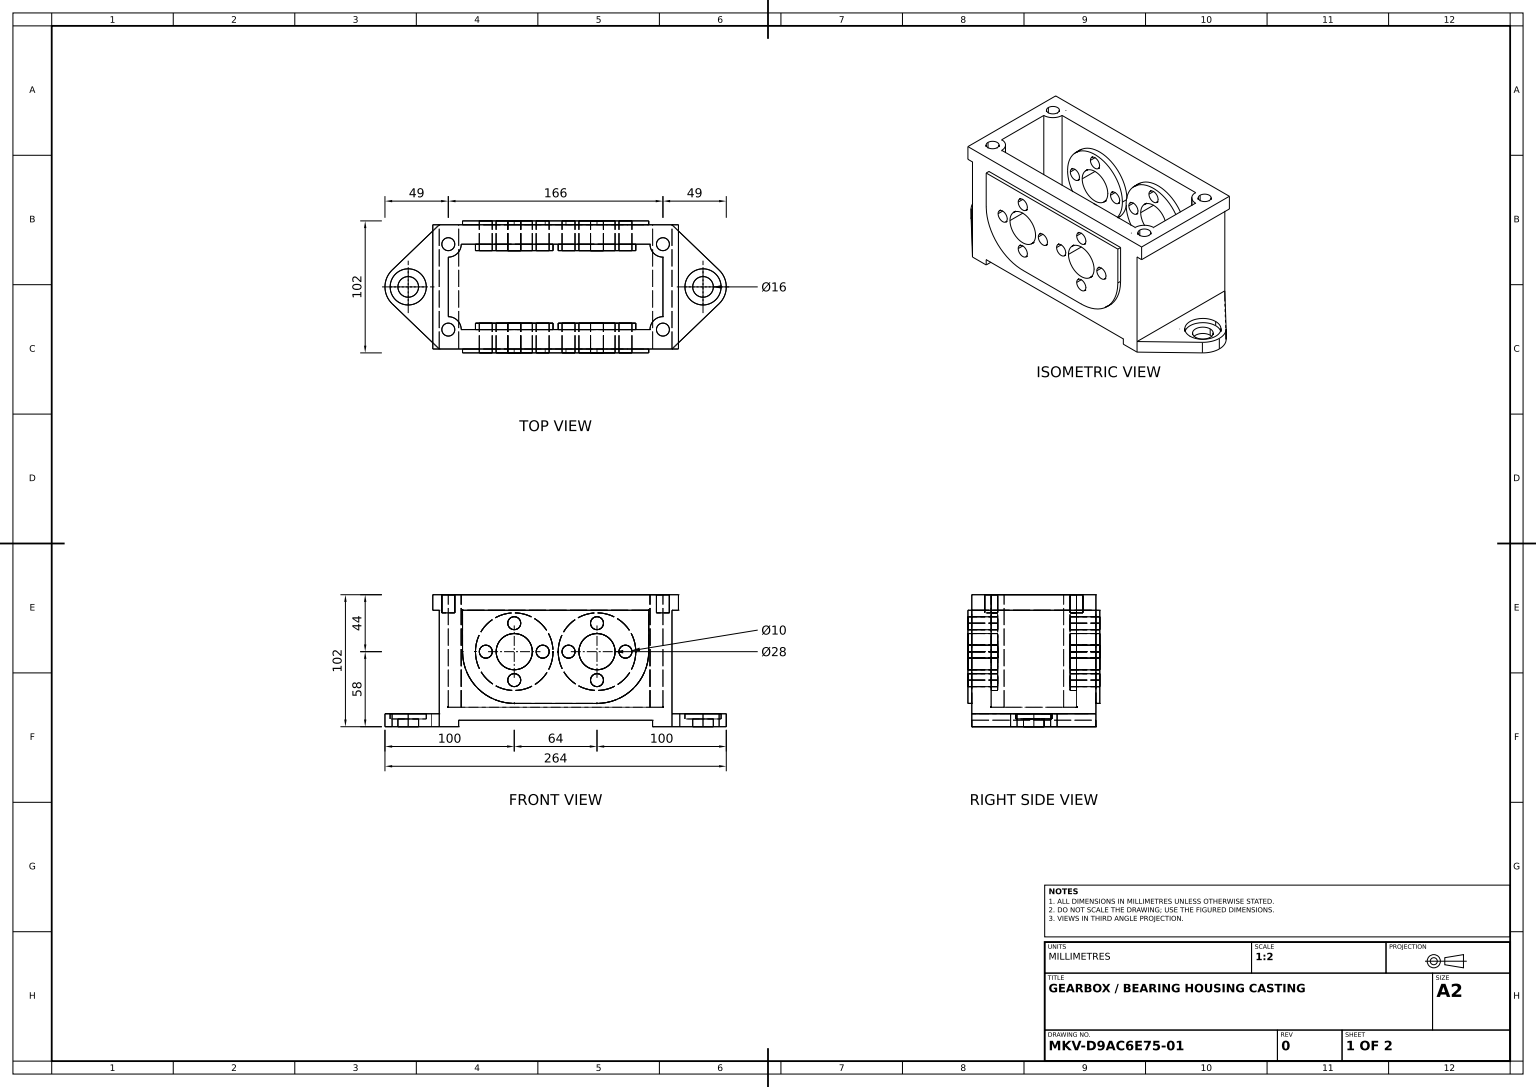
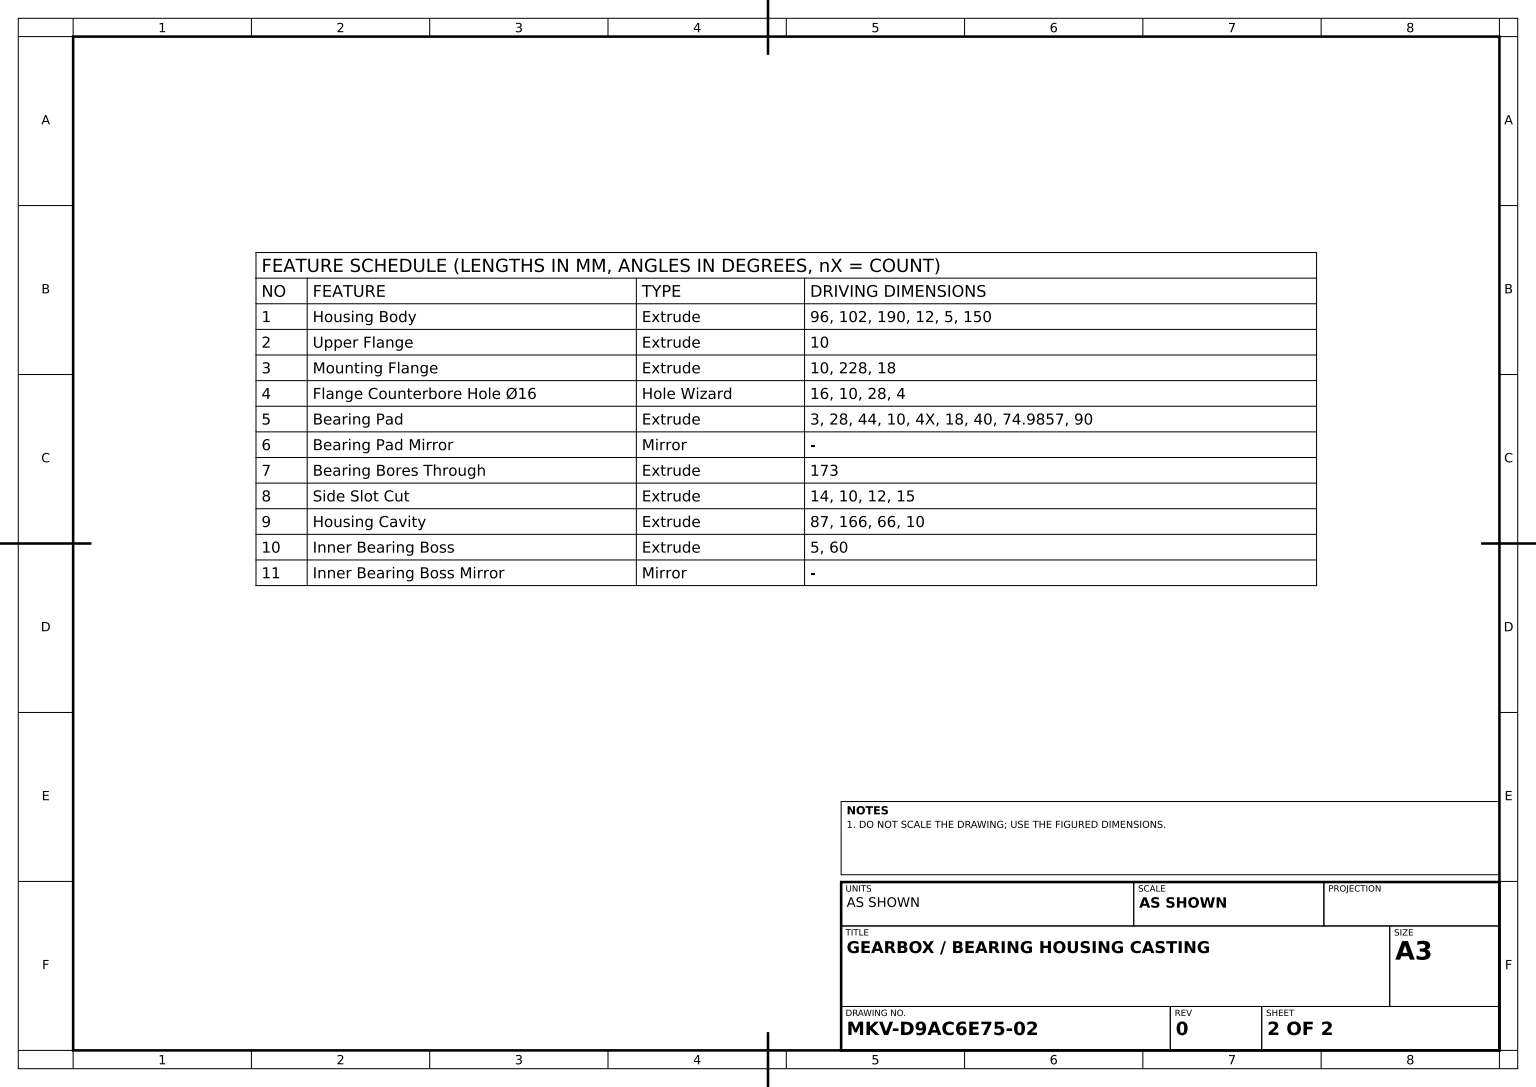
solid
v1 (75,-51,-48)
v2 (90,-51,-48)
e1 v1 v2 LINE
v3 (126.46707,-51,-12.983535)
e2 v2 v3 LINE
v4 (132,-51,0)
e3 v3 v4 CIRCLE(AX(P(114,-51,0),D(0,-1,0),D(1,0,0)),18)
v5 (126.46707,-51,12.983535)
e4 v4 v5 CIRCLE(AX(P(114,-51,0),D(0,-1,0),D(1,0,0)),18)
v6 (90,-51,48)
e5 v5 v6 LINE
v7 (75,-51,48)
e6 v7 v6 LINE
e7 v7 v1 LINE
v8 (114,-51,8)
v9 (114,-51,-8)
e8 v8 v9 CIRCLE(AX(P(114,-51,0),D(0,1,0),D(0,0,1)),8)
e9 v9 v8 CIRCLE(AX(P(114,-51,0),D(0,1,0),D(0,0,1)),8)
face PLANE(AX(P(0,-51,48),D(0,1,0),D(-1,0,0))) rev [e1 e2 e3 e4 e5 -e6 e7] [e8 e9]
v10 (78,37,33)
v11 (78,51,33)
e10 v10 v11 LINE
v12 (88,51,33)
e11 v11 v12 CIRCLE(AX(P(83,51,33),D(0,1,0),D(-1,0,0)),5)
v13 (88,37,33)
e12 v13 v12 LINE
e13 v10 v13 CIRCLE(AX(P(83,37,33),D(0,1,0),D(-1,0,0)),5)
face CYL(AX(P(83,37,33),D(0,1,0),D(-1,0,0)),5) rev [e10 e11 -e12 -e13]
v14 (-15,7,-51)
v15 (-5,7,-51)
e14 v14 v15 CIRCLE(AX(P(-10,7,-51),D(0,0,1),D(1,0,0)),5)
v16 (-15,7,-28)
e15 v16 v14 LINE
v17 (-5,7,-28)
e16 v17 v16 CIRCLE(AX(P(-10,7,-28),D(0,0,-1),D(1,0,0)),5)
e17 v17 v15 LINE
face CYL(AX(P(-10,7,51),D(0,0,-1),D(-1,0,0)),5) rev [-e14 -e15 -e16 e17]
v18 (-75,-46,48)
v19 (-75,-46,-48)
e18 v18 v19 LINE
v20 (75,-46,-48)
e19 v19 v20 LINE
v21 (75,-46,48)
e20 v21 v20 LINE
e21 v18 v21 LINE
face PLANE(AX(P(0,-46,48),D(0,1,0),D(-1,0,0))) rev [e18 e19 -e20 -e21]
v22 (-27,29,51)
v23 (-27,29,28)
e22 v22 v23 LINE
v24 (-37,29,51)
e23 v22 v24 CIRCLE(AX(P(-32,29,51),D(0,0,1),D(1,0,0)),5)
v25 (-37,29,28)
e24 v24 v25 LINE
e25 v25 v23 CIRCLE(AX(P(-32,29,28),D(0,0,-1),D(1,0,0)),5)
face CYL(AX(P(-32,29,51),D(0,0,-1),D(-1,0,0)),5) rev [-e22 e23 e24 e25]
v26 (2,7,28)
v27 (2,7,33)
e26 v26 v27 LINE
v28 (62,7,28)
e27 v28 v26 CIRCLE(AX(P(32,7,28),D(0,0,-1),D(-1,0,0)),30)
v29 (62,7,33)
e28 v28 v29 LINE
e29 v29 v27 CIRCLE(AX(P(32,7,33),D(0,0,-1),D(1,0,0)),30)
face CYL(AX(P(32,7,28),D(0,0,1),D(1,0,0)),30) [-e26 -e27 e28 e29]
v30 (-5,7,28)
v31 (-15,7,28)
e30 v30 v31 CIRCLE(AX(P(-10,7,28),D(0,0,-1),D(1,0,0)),5)
v32 (-15,7,51)
e31 v32 v31 LINE
v33 (-5,7,51)
e32 v32 v33 CIRCLE(AX(P(-10,7,51),D(0,0,1),D(1,0,0)),5)
e33 v33 v30 LINE
face CYL(AX(P(-10,7,51),D(0,0,-1),D(-1,0,0)),5) rev [e30 -e31 e32 e33]
v34 (72,7,51)
v35 (72,7,48)
e34 v34 v35 LINE
v36 (72,39,48)
e35 v35 v36 LINE
v37 (72,39,51)
e36 v37 v36 LINE
e37 v34 v37 LINE
face PLANE(AX(P(72,0,51),D(-1,0,0),D(0,0,1))) rev [e34 e35 -e36 -e37]
v38 (15,7,-51)
v39 (5,7,-51)
e38 v38 v39 CIRCLE(AX(P(10,7,-51),D(0,0,-1),D(1,0,0)),5)
v40 (5,7,-28)
e39 v40 v39 LINE
v41 (15,7,-28)
e40 v41 v40 CIRCLE(AX(P(10,7,-28),D(0,0,-1),D(-1,0,0)),5)
e41 v41 v38 LINE
face CYL(AX(P(10,7,51),D(0,0,-1),D(-1,0,0)),5) rev [e38 -e39 -e40 e41]
v42 (-18,7,28)
v43 (-46,7,28)
e42 v42 v43 CIRCLE(AX(P(-32,7,28),D(0,0,-1),D(1,0,0)),14)
v44 (-46,7,51)
e43 v44 v43 LINE
v45 (-18,7,51)
e44 v44 v45 CIRCLE(AX(P(-32,7,51),D(0,0,1),D(1,0,0)),14)
e45 v45 v42 LINE
face CYL(AX(P(-32,7,51),D(0,0,-1),D(-1,0,0)),14) rev [e42 -e43 e44 e45]
e46 v39 v38 CIRCLE(AX(P(10,7,-51),D(0,0,-1),D(1,0,0)),5)
e47 v40 v41 CIRCLE(AX(P(10,7,-28),D(0,0,-1),D(-1,0,0)),5)
face CYL(AX(P(10,7,51),D(0,0,-1),D(-1,0,0)),5) rev [e39 e46 -e41 -e47]
e48 v16 v17 CIRCLE(AX(P(-10,7,-28),D(0,0,-1),D(1,0,0)),5)
e49 v15 v14 CIRCLE(AX(P(-10,7,-51),D(0,0,1),D(1,0,0)),5)
face CYL(AX(P(-10,7,51),D(0,0,-1),D(-1,0,0)),5) rev [-e17 -e48 e15 -e49]
v46 (-37,-15,-28)
v47 (-27,-15,-28)
e50 v46 v47 CIRCLE(AX(P(-32,-15,-28),D(0,0,-1),D(1,0,0)),5)
v48 (-37,-15,-51)
e51 v46 v48 LINE
v49 (-27,-15,-51)
e52 v49 v48 CIRCLE(AX(P(-32,-15,-51),D(0,0,1),D(1,0,0)),5)
e53 v47 v49 LINE
face CYL(AX(P(-32,-15,51),D(0,0,-1),D(-1,0,0)),5) rev [-e50 e51 -e52 -e53]
v50 (114,-45,8)
e54 v8 v50 LINE
v51 (114,-45,-8)
e55 v50 v51 CIRCLE(AX(P(114,-45,0),D(0,1,0),D(0,0,1)),8)
e56 v9 v51 LINE
face CYL(AX(P(114,-41,0),D(0,1,0),D(0,0,1)),8) rev [e54 e55 -e56 -e8]
v52 (-83,-36,23)
v53 (-73,-36,33)
e57 v52 v53 CIRCLE(AX(P(-83,-36,33),D(0,-1,0),D(-1,0,0)),10)
v54 (73,-36,33)
e58 v53 v54 LINE
v55 (83,-36,23)
e59 v54 v55 CIRCLE(AX(P(83,-36,33),D(0,-1,0),D(-1,0,0)),10)
v56 (83,-36,-23)
e60 v55 v56 LINE
v57 (73,-36,-33)
e61 v56 v57 CIRCLE(AX(P(83,-36,-33),D(0,-1,0),D(-1,0,0)),10)
v58 (-73,-36,-33)
e62 v57 v58 LINE
v59 (-83,-36,-23)
e63 v58 v59 CIRCLE(AX(P(-83,-36,-33),D(0,-1,0),D(-1,0,0)),10)
e64 v59 v52 LINE
face PLANE(AX(P(-83,-36,33),D(0,1,0),D(-1,0,0))) [e57 e58 e59 e60 e61 e62 e63 e64]
v60 (-27,29,-51)
v61 (-37,29,-51)
e65 v60 v61 CIRCLE(AX(P(-32,29,-51),D(0,0,1),D(1,0,0)),5)
v62 (-27,29,-28)
e66 v62 v60 LINE
v63 (-37,29,-28)
e67 v63 v62 CIRCLE(AX(P(-32,29,-28),D(0,0,-1),D(1,0,0)),5)
e68 v63 v61 LINE
face CYL(AX(P(-32,29,51),D(0,0,-1),D(-1,0,0)),5) rev [-e65 -e66 -e67 e68]
v64 (-114,-51,8)
v65 (-114,-51,-8)
e69 v64 v65 CIRCLE(AX(P(-114,-51,0),D(0,1,0),D(0,0,1)),8)
e70 v65 v64 CIRCLE(AX(P(-114,-51,0),D(0,1,0),D(0,0,1)),8)
v66 (-126.46707,-51,12.983535)
v67 (-90,-51,48)
e71 v66 v67 LINE
v68 (-126.46707,-51,-12.983535)
e72 v66 v68 CIRCLE(AX(P(-114,-51,0),D(0,-1,0),D(0,0,-1)),18)
v69 (-90,-51,-48)
e73 v68 v69 LINE
v70 (-75,-51,-48)
e74 v69 v70 LINE
v71 (-75,-51,48)
e75 v71 v70 LINE
e76 v67 v71 LINE
face PLANE(AX(P(0,-51,48),D(0,1,0),D(0,0,1))) rev [e69 e70] [-e71 e72 e73 e74 -e75 -e76]
v72 (-37,-15,51)
v73 (-27,-15,51)
e77 v72 v73 CIRCLE(AX(P(-32,-15,51),D(0,0,1),D(1,0,0)),5)
v74 (-27,-15,28)
e78 v73 v74 LINE
v75 (-37,-15,28)
e79 v74 v75 CIRCLE(AX(P(-32,-15,28),D(0,0,-1),D(1,0,0)),5)
e80 v72 v75 LINE
face CYL(AX(P(-32,-15,51),D(0,0,-1),D(-1,0,0)),5) rev [e77 e78 e79 -e80]
v76 (15,7,51)
v77 (5,7,51)
e81 v76 v77 CIRCLE(AX(P(10,7,51),D(0,0,-1),D(1,0,0)),5)
v78 (15,7,28)
e82 v76 v78 LINE
v79 (5,7,28)
e83 v78 v79 CIRCLE(AX(P(10,7,28),D(0,0,-1),D(-1,0,0)),5)
e84 v77 v79 LINE
face CYL(AX(P(10,7,51),D(0,0,-1),D(-1,0,0)),5) rev [-e81 e82 e83 -e84]
e85 v45 v44 CIRCLE(AX(P(-32,7,51),D(0,0,1),D(1,0,0)),14)
e86 v43 v42 CIRCLE(AX(P(-32,7,28),D(0,0,-1),D(1,0,0)),14)
face CYL(AX(P(-32,7,51),D(0,0,-1),D(-1,0,0)),14) rev [e85 e43 e86 -e45]
v80 (37,29,28)
v81 (27,29,28)
e87 v80 v81 CIRCLE(AX(P(32,29,28),D(0,0,-1),D(-1,0,0)),5)
e88 v81 v80 CIRCLE(AX(P(32,29,28),D(0,0,-1),D(-1,0,0)),5)
v82 (37,-15,28)
v83 (27,-15,28)
e89 v82 v83 CIRCLE(AX(P(32,-15,28),D(0,0,-1),D(-1,0,0)),5)
e90 v83 v82 CIRCLE(AX(P(32,-15,28),D(0,0,-1),D(-1,0,0)),5)
v84 (18,7,28)
v85 (46,7,28)
e91 v84 v85 CIRCLE(AX(P(32,7,28),D(0,0,-1),D(-1,0,0)),14)
e92 v85 v84 CIRCLE(AX(P(32,7,28),D(0,0,-1),D(-1,0,0)),14)
e93 v26 v28 CIRCLE(AX(P(32,7,28),D(0,0,-1),D(-1,0,0)),30)
e94 v79 v78 CIRCLE(AX(P(10,7,28),D(0,0,-1),D(-1,0,0)),5)
v86 (59,7,28)
v87 (49,7,28)
e95 v86 v87 CIRCLE(AX(P(54,7,28),D(0,0,-1),D(-1,0,0)),5)
e96 v87 v86 CIRCLE(AX(P(54,7,28),D(0,0,-1),D(-1,0,0)),5)
face PLANE(AX(P(32,7,28),D(0,0,-1),D(-1,0,0))) [-e87 -e88] [-e89 -e90] [-e91 -e92] [e93 e27] [-e94 -e83] [-e95 -e96]
v88 (-114,-45,8)
e97 v64 v88 LINE
v89 (-114,-45,-8)
e98 v65 v89 LINE
e99 v89 v88 CIRCLE(AX(P(-114,-45,0),D(0,1,0),D(0,0,1)),8)
face CYL(AX(P(-114,-41,0),D(0,1,0),D(0,0,1)),8) rev [-e97 -e70 e98 e99]
v90 (46,7,51)
e100 v90 v85 LINE
v91 (18,7,51)
e101 v91 v84 LINE
e102 v90 v91 CIRCLE(AX(P(32,7,51),D(0,0,-1),D(1,0,0)),14)
face CYL(AX(P(32,7,51),D(0,0,-1),D(-1,0,0)),14) rev [e100 e92 -e101 -e102]
v92 (-46,7,-28)
v93 (-46,7,-51)
e103 v92 v93 LINE
v94 (-18,7,-51)
e104 v94 v93 CIRCLE(AX(P(-32,7,-51),D(0,0,1),D(1,0,0)),14)
v95 (-18,7,-28)
e105 v95 v94 LINE
e106 v92 v95 CIRCLE(AX(P(-32,7,-28),D(0,0,-1),D(1,0,0)),14)
face CYL(AX(P(-32,7,51),D(0,0,-1),D(-1,0,0)),14) rev [e103 -e104 -e105 -e106]
v96 (90,-41,48)
v97 (90,-41,-48)
e107 v96 v97 LINE
v98 (126.46707,-41,12.983535)
e108 v98 v96 LINE
v99 (132,-41,0)
e109 v99 v98 CIRCLE(AX(P(114,-41,0),D(0,-1,0),D(1,0,0)),18)
v100 (126.46707,-41,-12.983535)
e110 v100 v99 CIRCLE(AX(P(114,-41,0),D(0,-1,0),D(1,0,0)),18)
e111 v97 v100 LINE
v101 (114,-41,14)
v102 (114,-41,-14)
e112 v101 v102 CIRCLE(AX(P(114,-41,0),D(0,1,0),D(0,0,1)),14)
e113 v102 v101 CIRCLE(AX(P(114,-41,0),D(0,1,0),D(0,0,1)),14)
face PLANE(AX(P(114,-41,0),D(0,-1,0),D(1,0,0))) rev [-e107 -e108 -e109 -e110 -e111] [-e112 -e113]
v103 (95,39,48)
v104 (95,39,-48)
e114 v103 v104 LINE
v105 (90,39,48)
e115 v103 v105 LINE
v106 (90,39,-48)
e116 v105 v106 LINE
e117 v104 v106 LINE
face PLANE(AX(P(0,39,48),D(0,-1,0),D(0,0,-1))) [-e114 e115 e116 -e117]
v107 (-78,37,-33)
v108 (-78,51,-33)
e118 v107 v108 LINE
v109 (-88,37,-33)
e119 v109 v107 CIRCLE(AX(P(-83,37,-33),D(0,1,0),D(-1,0,0)),5)
v110 (-88,51,-33)
e120 v109 v110 LINE
e121 v110 v108 CIRCLE(AX(P(-83,51,-33),D(0,1,0),D(-1,0,0)),5)
face CYL(AX(P(-83,37,-33),D(0,1,0),D(-1,0,0)),5) rev [-e118 -e119 e120 e121]
v111 (32,-33,51)
v112 (32,-33,48)
e122 v111 v112 LINE
e123 v35 v112 CIRCLE(AX(P(32,7,48),D(0,0,-1),D(1,0,0)),40)
e124 v34 v111 CIRCLE(AX(P(32,7,51),D(0,0,-1),D(1,0,0)),40)
face CYL(AX(P(32,7,51),D(0,0,-1),D(-1,0,0)),40) [e122 -e123 -e34 e124]
v113 (-95,39,-48)
v114 (-90,39,-48)
e125 v113 v114 LINE
v115 (-90,39,48)
e126 v115 v114 LINE
v116 (-95,39,48)
e127 v116 v115 LINE
e128 v116 v113 LINE
face PLANE(AX(P(0,39,48),D(0,1,0),D(0,0,1))) rev [e125 -e126 -e127 e128]
e129 v99 v4 LINE
e130 v98 v5 LINE
face CYL(AX(P(114,-41,0),D(0,-1,0),D(1,0,0)),18) [-e129 e109 e130 -e4]
v117 (83,51,-23)
e131 v56 v117 LINE
v118 (73,51,-33)
e132 v117 v118 CIRCLE(AX(P(83,51,-33),D(0,-1,0),D(-1,0,0)),10)
e133 v57 v118 LINE
face CYL(AX(P(83,-36,-33),D(0,1,0),D(-1,0,0)),10) [e131 e132 -e133 -e61]
v119 (-72,39,48)
e134 v36 v119 LINE
v120 (-72,39,51)
e135 v120 v119 LINE
e136 v37 v120 LINE
face PLANE(AX(P(0,39,51),D(0,-1,0),D(0,0,-1))) rev [e134 -e135 -e136 e36]
e137 v96 v6 LINE
face PLANE(AX(P(90,-41,48),D(0.692614977,0,0.721307489),D(0.721307489,0,-0.692614977))) [-e130 e108 e137 -e5]
e138 v77 v76 CIRCLE(AX(P(10,7,51),D(0,0,-1),D(1,0,0)),5)
face CYL(AX(P(10,7,51),D(0,0,-1),D(-1,0,0)),5) rev [e94 -e82 -e138 e84]
v121 (-83,51,-23)
v122 (-83,51,23)
e139 v121 v122 LINE
e140 v52 v122 LINE
e141 v59 v121 LINE
face PLANE(AX(P(-83,-36,-23),D(-1,0,0),D(0,0,1))) rev [e139 -e140 -e64 e141]
v123 (-59,7,-28)
v124 (-59,7,-51)
e142 v123 v124 LINE
v125 (-49,7,-51)
e143 v125 v124 CIRCLE(AX(P(-54,7,-51),D(0,0,1),D(1,0,0)),5)
v126 (-49,7,-28)
e144 v126 v125 LINE
e145 v123 v126 CIRCLE(AX(P(-54,7,-28),D(0,0,-1),D(1,0,0)),5)
face CYL(AX(P(-54,7,51),D(0,0,-1),D(-1,0,0)),5) rev [e142 -e143 -e144 -e145]
v127 (27,-15,-51)
v128 (37,-15,-51)
e146 v127 v128 CIRCLE(AX(P(32,-15,-51),D(0,0,-1),D(1,0,0)),5)
v129 (37,-15,-28)
e147 v129 v128 LINE
v130 (27,-15,-28)
e148 v130 v129 CIRCLE(AX(P(32,-15,-28),D(0,0,-1),D(-1,0,0)),5)
e149 v130 v127 LINE
face CYL(AX(P(32,-15,51),D(0,0,-1),D(-1,0,0)),5) rev [e146 -e147 -e148 e149]
e150 v23 v25 CIRCLE(AX(P(-32,29,28),D(0,0,-1),D(1,0,0)),5)
e151 v24 v22 CIRCLE(AX(P(-32,29,51),D(0,0,1),D(1,0,0)),5)
face CYL(AX(P(-32,29,51),D(0,0,-1),D(-1,0,0)),5) rev [e150 -e24 e151 e22]
e152 v100 v3 LINE
face CYL(AX(P(114,-41,0),D(0,-1,0),D(1,0,0)),18) [-e3 -e152 e110 e129]
e153 v71 v18 LINE
e154 v21 v7 LINE
e155 v105 v96 LINE
v131 (95,51,48)
e156 v131 v103 LINE
v132 (-95,51,48)
e157 v132 v131 LINE
e158 v132 v116 LINE
v133 (-90,-41,48)
e159 v115 v133 LINE
e160 v133 v67 LINE
v134 (-72,7,48)
e161 v134 v119 LINE
v135 (-32,-33,48)
e162 v135 v112 LINE
e163 v134 v135 CIRCLE(AX(P(-32,7,48),D(0,0,1),D(1,0,0)),40)
face PLANE(AX(P(0,0,48),D(0,0,1),D(1,0,0))) [e153 e21 e154 e6 -e137 -e155 -e115 -e156 -e157 e158 e127 e159 e160 e76] [e161 -e134 -e35 e123 -e162 -e163]
v136 (73,51,33)
v137 (83,51,23)
e164 v136 v137 CIRCLE(AX(P(83,51,33),D(0,-1,0),D(-1,0,0)),10)
e165 v55 v137 LINE
e166 v54 v136 LINE
face CYL(AX(P(83,-36,33),D(0,1,0),D(-1,0,0)),10) [e164 -e165 -e59 e166]
v138 (-2,7,28)
v139 (-2,7,33)
e167 v138 v139 LINE
v140 (-62,7,33)
e168 v139 v140 CIRCLE(AX(P(-32,7,33),D(0,0,-1),D(1,0,0)),30)
v141 (-62,7,28)
e169 v141 v140 LINE
e170 v138 v141 CIRCLE(AX(P(-32,7,28),D(0,0,-1),D(1,0,0)),30)
face CYL(AX(P(-32,7,28),D(0,0,1),D(1,0,0)),30) [e167 e168 -e169 -e170]
e171 v106 v97 LINE
face PLANE(AX(P(90,0,48),D(1,0,0),D(0,0,-1))) [e107 -e171 -e116 e155]
e172 v91 v90 CIRCLE(AX(P(32,7,51),D(0,0,-1),D(1,0,0)),14)
face CYL(AX(P(32,7,51),D(0,0,-1),D(-1,0,0)),14) rev [-e172 e101 e91 -e100]
v142 (59,7,51)
v143 (49,7,51)
e173 v142 v143 CIRCLE(AX(P(54,7,51),D(0,0,-1),D(1,0,0)),5)
e174 v142 v86 LINE
e175 v143 v87 LINE
face CYL(AX(P(54,7,51),D(0,0,-1),D(-1,0,0)),5) rev [-e173 e174 e95 -e175]
v144 (46,7,-28)
v145 (46,7,-51)
e176 v144 v145 LINE
v146 (18,7,-28)
e177 v146 v144 CIRCLE(AX(P(32,7,-28),D(0,0,-1),D(-1,0,0)),14)
v147 (18,7,-51)
e178 v146 v147 LINE
e179 v147 v145 CIRCLE(AX(P(32,7,-51),D(0,0,-1),D(1,0,0)),14)
face CYL(AX(P(32,7,51),D(0,0,-1),D(-1,0,0)),14) rev [-e176 -e177 e178 e179]
v148 (78,37,-33)
v149 (88,37,-33)
e180 v148 v149 CIRCLE(AX(P(83,37,-33),D(0,1,0),D(1,0,0)),5)
e181 v149 v148 CIRCLE(AX(P(83,37,-33),D(0,1,0),D(1,0,0)),5)
face PLANE(AX(P(83,37,-33),D(0,-1,0),D(1,0,0))) rev [e180 e181]
v150 (114,-45,-14)
v151 (114,-45,14)
e182 v150 v151 CIRCLE(AX(P(114,-45,0),D(0,1,0),D(0,0,1)),14)
e183 v151 v150 CIRCLE(AX(P(114,-45,0),D(0,1,0),D(0,0,1)),14)
e184 v51 v50 CIRCLE(AX(P(114,-45,0),D(0,1,0),D(0,0,1)),8)
face PLANE(AX(P(122,-45,0),D(0,-1,0),D(0,0,-1))) rev [e182 e183] [-e184 -e55]
e185 v124 v125 CIRCLE(AX(P(-54,7,-51),D(0,0,1),D(1,0,0)),5)
e186 v126 v123 CIRCLE(AX(P(-54,7,-28),D(0,0,-1),D(1,0,0)),5)
face CYL(AX(P(-54,7,51),D(0,0,-1),D(-1,0,0)),5) rev [e144 -e185 -e142 -e186]
v152 (-90,-41,-48)
e187 v114 v152 LINE
v153 (-95,51,-48)
e188 v153 v113 LINE
v154 (95,51,-48)
e189 v153 v154 LINE
e190 v154 v104 LINE
e191 v97 v2 LINE
e192 v20 v1 LINE
e193 v70 v19 LINE
e194 v152 v69 LINE
v155 (72,7,-48)
v156 (72,39,-48)
e195 v155 v156 LINE
v157 (-72,39,-48)
e196 v156 v157 LINE
v158 (-72,7,-48)
e197 v158 v157 LINE
v159 (-32,-33,-48)
e198 v158 v159 CIRCLE(AX(P(-32,7,-48),D(0,0,1),D(1,0,0)),40)
v160 (32,-33,-48)
e199 v159 v160 LINE
e200 v155 v160 CIRCLE(AX(P(32,7,-48),D(0,0,-1),D(1,0,0)),40)
face PLANE(AX(P(0,0,-48),D(0,0,1),D(1,0,0))) rev [-e187 -e125 -e188 e189 e190 e117 e171 e191 -e1 -e192 -e19 -e193 -e74 -e194] [e195 e196 -e197 e198 e199 -e200]
e201 v108 v110 CIRCLE(AX(P(-83,51,-33),D(0,1,0),D(-1,0,0)),5)
e202 v107 v109 CIRCLE(AX(P(-83,37,-33),D(0,1,0),D(-1,0,0)),5)
face CYL(AX(P(-83,37,-33),D(0,1,0),D(-1,0,0)),5) rev [e118 e201 -e120 -e202]
v161 (62,7,-33)
v162 (2,7,-33)
e203 v161 v162 CIRCLE(AX(P(32,7,-33),D(0,0,-1),D(-1,0,0)),30)
e204 v162 v161 CIRCLE(AX(P(32,7,-33),D(0,0,-1),D(-1,0,0)),30)
v163 (-2,7,-33)
v164 (-62,7,-33)
e205 v163 v164 CIRCLE(AX(P(-32,7,-33),D(0,0,-1),D(1,0,0)),30)
e206 v164 v163 CIRCLE(AX(P(-32,7,-33),D(0,0,-1),D(1,0,0)),30)
v165 (-73,51,-33)
e207 v58 v165 LINE
e208 v118 v165 LINE
face PLANE(AX(P(-73,-36,-33),D(0,0,-1),D(-1,0,0))) rev [e203 e204] [e205 e206] [-e207 -e62 e133 e208]
e209 v133 v152 LINE
face PLANE(AX(P(-90,0,48),D(1,0,0),D(0,0,-1))) rev [-e209 -e159 e126 e187]
v166 (37,29,-28)
v167 (37,29,-51)
e210 v166 v167 LINE
v168 (27,29,-51)
e211 v167 v168 CIRCLE(AX(P(32,29,-51),D(0,0,-1),D(1,0,0)),5)
v169 (27,29,-28)
e212 v169 v168 LINE
e213 v166 v169 CIRCLE(AX(P(32,29,-28),D(0,0,-1),D(-1,0,0)),5)
face CYL(AX(P(32,29,51),D(0,0,-1),D(-1,0,0)),5) rev [e210 e211 -e212 -e213]
v170 (27,29,51)
v171 (37,29,51)
e214 v170 v171 CIRCLE(AX(P(32,29,51),D(0,0,-1),D(1,0,0)),5)
e215 v171 v170 CIRCLE(AX(P(32,29,51),D(0,0,-1),D(1,0,0)),5)
e216 v143 v142 CIRCLE(AX(P(54,7,51),D(0,0,-1),D(1,0,0)),5)
v172 (-72,7,51)
e217 v172 v120 LINE
v173 (-32,-33,51)
e218 v172 v173 CIRCLE(AX(P(-32,7,51),D(0,0,1),D(1,0,0)),40)
e219 v173 v111 LINE
v174 (-49,7,51)
v175 (-59,7,51)
e220 v174 v175 CIRCLE(AX(P(-54,7,51),D(0,0,1),D(1,0,0)),5)
e221 v175 v174 CIRCLE(AX(P(-54,7,51),D(0,0,1),D(1,0,0)),5)
v176 (27,-15,51)
v177 (37,-15,51)
e222 v176 v177 CIRCLE(AX(P(32,-15,51),D(0,0,-1),D(1,0,0)),5)
e223 v177 v176 CIRCLE(AX(P(32,-15,51),D(0,0,-1),D(1,0,0)),5)
e224 v33 v32 CIRCLE(AX(P(-10,7,51),D(0,0,1),D(1,0,0)),5)
e225 v73 v72 CIRCLE(AX(P(-32,-15,51),D(0,0,1),D(1,0,0)),5)
face PLANE(AX(P(0,0,51),D(0,0,1),D(1,0,0))) [e138 e81] [e214 e215] [e173 e216] [e172 e102] [-e124 e37 e136 -e217 e218 e219] [-e44 -e85] [-e23 -e151] [-e220 -e221] [e222 e223] [-e32 -e224] [-e225 -e77]
e226 v141 v138 CIRCLE(AX(P(-32,7,28),D(0,0,-1),D(1,0,0)),30)
e227 v140 v139 CIRCLE(AX(P(-32,7,33),D(0,0,-1),D(1,0,0)),30)
face CYL(AX(P(-32,7,28),D(0,0,1),D(1,0,0)),30) [-e167 -e226 e169 e227]
v178 (-59,7,28)
v179 (-49,7,28)
e228 v178 v179 CIRCLE(AX(P(-54,7,28),D(0,0,-1),D(1,0,0)),5)
e229 v179 v178 CIRCLE(AX(P(-54,7,28),D(0,0,-1),D(1,0,0)),5)
e230 v75 v74 CIRCLE(AX(P(-32,-15,28),D(0,0,-1),D(1,0,0)),5)
e231 v31 v30 CIRCLE(AX(P(-10,7,28),D(0,0,-1),D(1,0,0)),5)
face PLANE(AX(P(-32,7,28),D(0,0,1),D(1,0,0))) rev [e226 e170] [-e150 -e25] [-e228 -e229] [-e79 -e230] [-e42 -e86] [-e231 -e30]
v180 (72,7,-51)
v181 (32,-33,-51)
e232 v180 v181 CIRCLE(AX(P(32,7,-51),D(0,0,-1),D(1,0,0)),40)
e233 v180 v155 LINE
e234 v181 v160 LINE
face CYL(AX(P(32,7,-51),D(0,0,1),D(1,0,0)),40) [-e232 e233 e200 -e234]
e235 v165 v121 CIRCLE(AX(P(-83,51,-33),D(0,-1,0),D(-1,0,0)),10)
face CYL(AX(P(-83,-36,-33),D(0,1,0),D(-1,0,0)),10) [-e63 e207 e235 -e141]
e236 v145 v147 CIRCLE(AX(P(32,7,-51),D(0,0,-1),D(1,0,0)),14)
e237 v144 v146 CIRCLE(AX(P(32,7,-28),D(0,0,-1),D(-1,0,0)),14)
face CYL(AX(P(32,7,51),D(0,0,-1),D(-1,0,0)),14) rev [e236 -e178 -e237 e176]
v182 (-126.46707,-41,12.983535)
v183 (-126.46707,-41,-12.983535)
e238 v182 v183 CIRCLE(AX(P(-114,-41,0),D(0,-1,0),D(0,0,-1)),18)
e239 v183 v68 LINE
e240 v182 v66 LINE
face CYL(AX(P(-114,-41,0),D(0,-1,0),D(0,0,-1)),18) [e238 e239 -e72 -e240]
e241 v172 v134 LINE
face PLANE(AX(P(-72,0,51),D(-1,0,0),D(0,0,1))) [-e161 -e241 e217 e135]
face PLANE(AX(P(75,0,48),D(1,0,0),D(0,1,0))) rev [-e154 e20 e192 -e7]
e242 v183 v152 LINE
face PLANE(AX(P(-126.46707,-41,-12.983535),D(-0.692614977,0,-0.721307489),D(-0.721307489,0,0.692614977))) [-e239 e242 e194 -e73]
v184 (-72,39,-51)
e243 v184 v157 LINE
v185 (72,39,-51)
e244 v185 v156 LINE
e245 v185 v184 LINE
face PLANE(AX(P(0,39,-51),D(0,1,0),D(0,0,1))) [e243 -e196 -e244 e245]
v186 (49,7,-28)
v187 (59,7,-28)
e246 v186 v187 CIRCLE(AX(P(54,7,-28),D(0,0,-1),D(-1,0,0)),5)
e247 v187 v186 CIRCLE(AX(P(54,7,-28),D(0,0,-1),D(-1,0,0)),5)
e248 v129 v130 CIRCLE(AX(P(32,-15,-28),D(0,0,-1),D(-1,0,0)),5)
v188 (62,7,-28)
v189 (2,7,-28)
e249 v188 v189 CIRCLE(AX(P(32,7,-28),D(0,0,-1),D(-1,0,0)),30)
e250 v189 v188 CIRCLE(AX(P(32,7,-28),D(0,0,-1),D(-1,0,0)),30)
e251 v169 v166 CIRCLE(AX(P(32,29,-28),D(0,0,-1),D(-1,0,0)),5)
face PLANE(AX(P(32,7,-28),D(0,0,1),D(-1,0,0))) [e246 e247] [e148 e248] [-e249 -e250] [e177 e237] [e40 e47] [e251 e213]
v190 (-73,51,33)
e252 v53 v190 LINE
e253 v190 v136 LINE
e254 v27 v29 CIRCLE(AX(P(32,7,33),D(0,0,-1),D(1,0,0)),30)
face PLANE(AX(P(-73,-36,33),D(0,0,1),D(1,0,0))) rev [e252 e253 -e166 -e58] [-e168 -e227] [-e254 -e29]
v191 (-88,37,33)
v192 (-78,37,33)
e255 v191 v192 CIRCLE(AX(P(-83,37,33),D(0,1,0),D(1,0,0)),5)
v193 (-88,51,33)
e256 v191 v193 LINE
v194 (-78,51,33)
e257 v193 v194 CIRCLE(AX(P(-83,51,33),D(0,1,0),D(1,0,0)),5)
e258 v192 v194 LINE
face CYL(AX(P(-83,37,33),D(0,1,0),D(-1,0,0)),5) rev [-e255 e256 e257 -e258]
e259 v13 v10 CIRCLE(AX(P(83,37,33),D(0,1,0),D(-1,0,0)),5)
e260 v12 v11 CIRCLE(AX(P(83,51,33),D(0,1,0),D(-1,0,0)),5)
face CYL(AX(P(83,37,33),D(0,1,0),D(-1,0,0)),5) rev [-e10 -e259 e12 e260]
face CYL(AX(P(-32,-15,51),D(0,0,-1),D(-1,0,0)),5) rev [e80 e230 -e78 e225]
e261 v137 v117 LINE
e262 v122 v190 CIRCLE(AX(P(-83,51,33),D(0,-1,0),D(-1,0,0)),10)
e263 v194 v193 CIRCLE(AX(P(-83,51,33),D(0,1,0),D(1,0,0)),5)
e264 v132 v153 LINE
e265 v131 v154 LINE
v195 (78,51,-33)
v196 (88,51,-33)
e266 v195 v196 CIRCLE(AX(P(83,51,-33),D(0,1,0),D(1,0,0)),5)
e267 v196 v195 CIRCLE(AX(P(83,51,-33),D(0,1,0),D(1,0,0)),5)
face PLANE(AX(P(0,51,48),D(0,1,0),D(-1,0,0))) [-e235 -e208 -e132 -e261 -e164 -e253 -e262 -e139] [-e257 -e263] [-e264 e157 e265 -e189] [-e266 -e267] [-e260 -e11] [-e121 -e201]
v197 (-114,-45,-14)
v198 (-114,-45,14)
e268 v197 v198 CIRCLE(AX(P(-114,-45,0),D(0,1,0),D(0,0,1)),14)
v199 (-114,-41,-14)
e269 v197 v199 LINE
v200 (-114,-41,14)
e270 v199 v200 CIRCLE(AX(P(-114,-41,0),D(0,1,0),D(0,0,1)),14)
e271 v198 v200 LINE
face CYL(AX(P(-114,-41,0),D(0,1,0),D(0,0,1)),14) rev [-e268 e269 e270 -e271]
face PLANE(AX(P(-75,0,48),D(-1,0,0),D(0,0,1))) rev [e75 e193 -e18 -e153]
v201 (-2,7,-28)
v202 (-62,7,-28)
e272 v201 v202 CIRCLE(AX(P(-32,7,-28),D(0,0,-1),D(1,0,0)),30)
e273 v202 v164 LINE
e274 v201 v163 LINE
face CYL(AX(P(-32,7,-28),D(0,0,-1),D(-1,0,0)),30) [e272 e273 -e205 -e274]
face PLANE(AX(P(83,37,33),D(0,1,0),D(-1,0,0))) [e259 e13]
face CYL(AX(P(32,7,28),D(0,0,1),D(1,0,0)),30) [-e28 -e93 e26 e254]
e275 v171 v80 LINE
e276 v170 v81 LINE
face CYL(AX(P(32,29,51),D(0,0,-1),D(-1,0,0)),5) rev [e88 -e275 -e214 e276]
v203 (59,7,-51)
e277 v187 v203 LINE
v204 (49,7,-51)
e278 v203 v204 CIRCLE(AX(P(54,7,-51),D(0,0,-1),D(1,0,0)),5)
e279 v186 v204 LINE
face CYL(AX(P(54,7,51),D(0,0,-1),D(-1,0,0)),5) rev [e277 e278 -e279 -e247]
e280 v202 v201 CIRCLE(AX(P(-32,7,-28),D(0,0,-1),D(1,0,0)),30)
face CYL(AX(P(-32,7,-28),D(0,0,-1),D(-1,0,0)),30) [e274 -e206 -e273 e280]
face PLANE(AX(P(90,-41,-48),D(0.692614977,0,-0.721307489),D(-0.721307489,0,-0.692614977))) [-e2 -e191 e111 e152]
e281 v182 v133 LINE
face PLANE(AX(P(-126.46707,-41,12.983535),D(0.692614977,0,-0.721307489),D(-0.721307489,0,-0.692614977))) rev [-e281 e240 e71 -e160]
e282 v47 v46 CIRCLE(AX(P(-32,-15,-28),D(0,0,-1),D(1,0,0)),5)
e283 v48 v49 CIRCLE(AX(P(-32,-15,-51),D(0,0,1),D(1,0,0)),5)
face CYL(AX(P(-32,-15,51),D(0,0,-1),D(-1,0,0)),5) rev [-e51 -e282 e53 -e283]
e284 v95 v92 CIRCLE(AX(P(-32,7,-28),D(0,0,-1),D(1,0,0)),14)
e285 v93 v94 CIRCLE(AX(P(-32,7,-51),D(0,0,1),D(1,0,0)),14)
face CYL(AX(P(-32,7,51),D(0,0,-1),D(-1,0,0)),14) rev [-e103 -e284 e105 -e285]
e286 v173 v135 LINE
face PLANE(AX(P(0,-33,51),D(0,1,0),D(0,0,1))) rev [-e122 -e219 e286 e162]
e287 v177 v82 LINE
e288 v176 v83 LINE
face CYL(AX(P(32,-15,51),D(0,0,-1),D(-1,0,0)),5) rev [e90 -e287 -e222 e288]
face CYL(AX(P(-83,-36,33),D(0,1,0),D(-1,0,0)),10) [e262 -e252 -e57 e140]
v205 (-72,7,-51)
e289 v205 v184 LINE
e290 v205 v158 LINE
face PLANE(AX(P(-72,0,-51),D(1,0,0),D(0,0,-1))) rev [e197 -e243 -e289 e290]
e291 v200 v199 CIRCLE(AX(P(-114,-41,0),D(0,1,0),D(0,0,1)),14)
face PLANE(AX(P(-114,-41,0),D(0,-1,0),D(0,0,-1))) rev [-e291 -e270] [e209 -e242 -e238 e281]
e292 v180 v185 LINE
face PLANE(AX(P(72,0,-51),D(1,0,0),D(0,0,-1))) [e292 e244 -e195 -e233]
e293 v198 v197 CIRCLE(AX(P(-114,-45,0),D(0,1,0),D(0,0,1)),14)
face CYL(AX(P(-114,-41,0),D(0,1,0),D(0,0,1)),14) rev [e271 e291 -e269 -e293]
e294 v128 v127 CIRCLE(AX(P(32,-15,-51),D(0,0,-1),D(1,0,0)),5)
face CYL(AX(P(32,-15,51),D(0,0,-1),D(-1,0,0)),5) rev [-e149 -e248 e147 e294]
face CYL(AX(P(114,-41,0),D(0,1,0),D(0,0,1)),8) rev [-e9 e56 e184 -e54]
face CYL(AX(P(32,29,51),D(0,0,-1),D(-1,0,0)),5) rev [-e215 e275 e87 -e276]
e295 v192 v191 CIRCLE(AX(P(-83,37,33),D(0,1,0),D(1,0,0)),5)
face PLANE(AX(P(-83,37,33),D(0,-1,0),D(1,0,0))) rev [e295 e255]
face PLANE(AX(P(83,-36,-23),D(1,0,0),D(0,0,-1))) rev [-e131 -e60 e165 e261]
e296 v168 v167 CIRCLE(AX(P(32,29,-51),D(0,0,-1),D(1,0,0)),5)
face CYL(AX(P(32,29,51),D(0,0,-1),D(-1,0,0)),5) rev [e296 -e210 -e251 e212]
face PLANE(AX(P(-83,37,-33),D(0,1,0),D(-1,0,0))) [e202 e119]
face CYL(AX(P(-32,7,51),D(0,0,-1),D(-1,0,0)),40) [-e286 -e218 e241 e163]
e297 v204 v203 CIRCLE(AX(P(54,7,-51),D(0,0,-1),D(1,0,0)),5)
face CYL(AX(P(54,7,51),D(0,0,-1),D(-1,0,0)),5) rev [-e277 -e246 e279 e297]
e298 v61 v60 CIRCLE(AX(P(-32,29,-51),D(0,0,1),D(1,0,0)),5)
e299 v62 v63 CIRCLE(AX(P(-32,29,-28),D(0,0,-1),D(1,0,0)),5)
face CYL(AX(P(-32,29,51),D(0,0,-1),D(-1,0,0)),5) rev [-e298 -e68 -e299 e66]
v206 (-32,-33,-51)
e300 v206 v159 LINE
e301 v206 v181 LINE
face PLANE(AX(P(0,-33,-51),D(0,-1,0),D(0,0,-1))) [-e199 -e300 e301 e234]
e302 v88 v89 CIRCLE(AX(P(-114,-45,0),D(0,1,0),D(0,0,1)),8)
face PLANE(AX(P(-106,-45,0),D(0,-1,0),D(0,0,-1))) rev [e293 e268] [-e302 -e99]
e303 v150 v102 LINE
e304 v151 v101 LINE
face CYL(AX(P(114,-41,0),D(0,1,0),D(0,0,1)),14) rev [e112 -e303 -e183 e304]
e305 v149 v196 LINE
e306 v148 v195 LINE
face CYL(AX(P(83,37,-33),D(0,1,0),D(-1,0,0)),5) rev [e305 e267 -e306 -e181]
face CYL(AX(P(-114,-41,0),D(0,1,0),D(0,0,1)),8) rev [-e98 -e69 e97 e302]
face PLANE(AX(P(-32,7,-28),D(0,0,-1),D(1,0,0))) rev [e106 e284] [e67 e299] [e186 e145] [-e272 -e280] [e282 e50] [e48 e16]
face CYL(AX(P(-10,7,51),D(0,0,-1),D(-1,0,0)),5) rev [e31 e231 -e33 e224]
e307 v205 v206 CIRCLE(AX(P(-32,7,-51),D(0,0,1),D(1,0,0)),40)
face CYL(AX(P(-32,7,-51),D(0,0,1),D(1,0,0)),40) [e300 -e198 -e290 e307]
face PLANE(AX(P(-95,0,48),D(1,0,0),D(0,0,-1))) rev [e264 e188 -e128 -e158]
e308 v188 v161 LINE
e309 v189 v162 LINE
face CYL(AX(P(32,7,-28),D(0,0,-1),D(-1,0,0)),30) [-e308 e249 e309 -e203]
face CYL(AX(P(-83,37,33),D(0,1,0),D(-1,0,0)),5) rev [e263 -e256 -e295 e258]
face PLANE(AX(P(95,0,48),D(1,0,0),D(0,0,-1))) [e156 e114 -e190 -e265]
face CYL(AX(P(54,7,51),D(0,0,-1),D(-1,0,0)),5) rev [-e174 -e216 e175 e96]
e310 v174 v179 LINE
e311 v175 v178 LINE
face CYL(AX(P(-54,7,51),D(0,0,-1),D(-1,0,0)),5) rev [e310 e229 -e311 e221]
face CYL(AX(P(32,-15,51),D(0,0,-1),D(-1,0,0)),5) rev [e287 e89 -e288 -e223]
face CYL(AX(P(114,-41,0),D(0,1,0),D(0,0,1)),14) rev [-e304 -e182 e303 e113]
face PLANE(AX(P(0,0,-51),D(0,0,-1),D(1,0,0))) [-e278 -e297] [e52 e283] [-e179 -e236] [-e211 -e296] [e285 e104] [e49 e14] [e185 e143] [-e46 -e38] [-e294 -e146] [-e292 e232 -e301 -e307 e289 -e245] [e298 e65]
face CYL(AX(P(83,37,-33),D(0,1,0),D(-1,0,0)),5) rev [e266 -e305 -e180 e306]
face CYL(AX(P(-54,7,51),D(0,0,-1),D(-1,0,0)),5) rev [e228 -e310 e220 e311]
face CYL(AX(P(32,7,-28),D(0,0,-1),D(-1,0,0)),30) [e250 e308 -e204 -e309]
